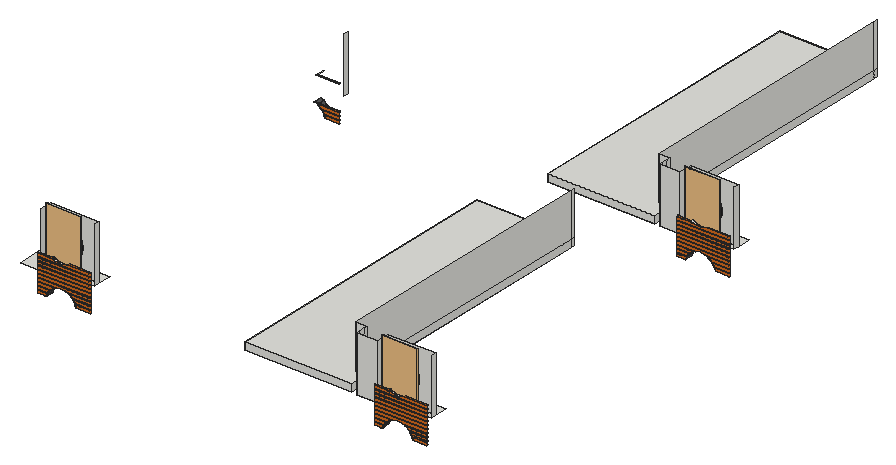
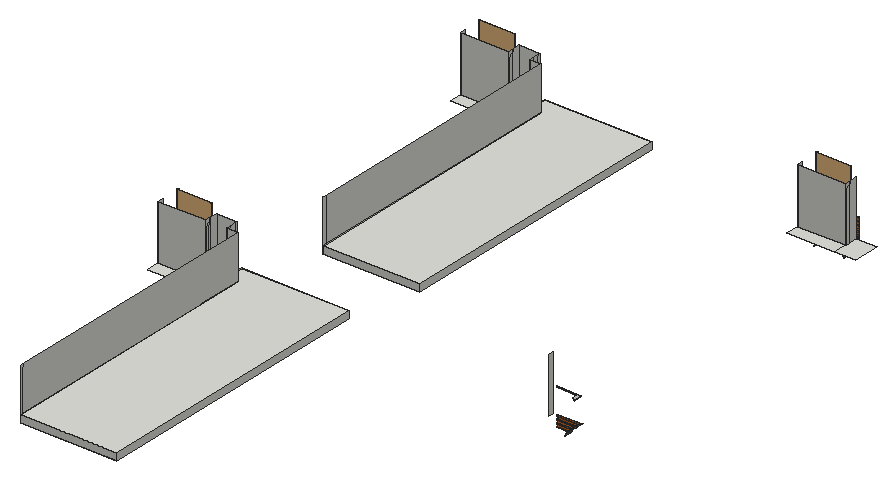
# SketchUp Ruby script. Lengths in inches.
U = 1.inch
M = Sketchup.active_model
def pt(a) = Geom::Point3d.new(a.map { |v| v * U })
def face(e, loops, mat)
  f = e.add_face(loops[0].map { |a| pt(a) })
  loops[1..].each { |l| e.add_face(l.map { |a| pt(a) }).erase! }
  f.material = f.back_material = mat if mat
  f
end
# faces: each face lists its corners as indices into pts; further lists are holes
def faces(e, pts, list, mat = nil) = list.each { |f| face(e, (f[0].is_a?(Array) ? f : [f]).map { |l| l.map { |i| pts[i] } }, mat) }
# xy, xz, yz: faces in a plane at the given z, y or x. An outline is a flat list of corners, or four numbers for a rectangle; further outlines are holes
def ring(l) = l.size == 4 ? [[l[0], l[1]], [l[2], l[1]], [l[2], l[3]], [l[0], l[3]]] : l.each_slice(2).to_a
def flat(e, list, mat, &to3) = list.each { |f| face(e, (f[0].is_a?(Array) ? f : [f]).map { |l| ring(l).map { |u, v| to3.(u, v) } }, mat) }
def xy(e, z, list, mat = nil) = flat(e, list, mat) { |x, y| [x, y, z] }
def xz(e, y, list, mat = nil) = flat(e, list, mat) { |x, z| [x, y, z] }
def yz(e, x, list, mat = nil) = flat(e, list, mat) { |y, z| [x, y, z] }
def lines(e, pts, list) = list.each { |a, b| e.add_line(pt(pts[a]), pt(pts[b])) }
# prism: a flat outline (further loops are holes) pulled along v
def prism(e, loops, v, mat = nil)
  f = face(e, loops, mat); d = Geom::Vector3d.new(v.map { |x| x * U })
  f.pushpull(f.normal.samedirection?(d) ? d.length : -d.length)
end
def box(e, o, s, mat = nil) = prism(e, [[o, [o[0] + s[0], o[1], o[2]], [o[0] + s[0], o[1] + s[1], o[2]], [o[0], o[1] + s[1], o[2]]]], [0, 0, s[2]], mat)
def at(x, y, z, deg = 0) = Geom::Transformation.translation(pt([x, y, z])) * Geom::Transformation.rotation(ORIGIN, Z_AXIS, deg.degrees)
def axes(o, x, y, z) = Geom::Transformation.new([*x, 0, *y, 0, *z, 0, *pt(o).to_a, 1])
def part(name) = M.definitions.add(name)
# library, detail: a bought-in or finely detailed component or shape, given as its bounding box
def library(name, o, s) = part(name).tap { |d| box(d.entities, o, s) }
def detail(e, o, s) = box(e.add_group.entities, o, s)
def put(e, d, t, mat = nil) = e.add_instance(d, t).tap { |i| i.material = mat if mat }
def group(e, t, mat = nil) = e.add_group.tap { |g| g.transformation = t; g.material = mat if mat }.entities
root = M.entities
M.materials.add("[0041_Chocolate]").color = [210, 105, 30]
M.materials.add("[Color M06]").color = [84, 84, 84]
M.materials.add("[Color M08]").color = [30, 30, 30]
c1 = library("1",[3.97,34.78,0],[101.43,33.99,0.79])
xy(root,260.375,[[1547.711,280.466,1564.025,281.466],[1621.742,280.466,1649.144,281.466],[2198.211,280.466,2214.525,281.466],[2272.242,280.466,2299.644,281.466],[1550.055,971.36,1577.456,972.36],
  [2230.648,971.36,2246.963,972.36],[2304.68,971.36,2332.081,972.36]],"[0041_Chocolate]")
xy(root,265.329,[[1547.711,280.466,1565.895,281.466],[1619.873,280.466,1649.144,281.466],[2198.211,280.466,2216.395,281.466],[2270.373,280.466,2299.644,281.466],[1548.185,971.36,1577.456,972.36],
  [2230.648,971.36,2248.832,972.36],[2302.81,971.36,2332.081,972.36]],"[0041_Chocolate]")
xy(root,267.4375,[[1547.711,280.466,1566.768,281.466],[1619,280.466,1649.144,281.466],[2198.211,280.466,2217.268,281.466],[2269.5,280.466,2299.644,281.466],[1547.312,971.36,1577.456,972.36],
  [2230.648,971.36,2249.705,972.36],[2301.937,971.36,2332.081,972.36]],"[0041_Chocolate]")
xy(root,272.392,[[1547.711,280.466,1570.298,281.466],[1615.47,280.466,1649.144,281.466],[2198.211,280.466,2220.798,281.466],[2265.97,280.466,2299.644,281.466],[1543.782,971.36,1577.456,972.36],
  [2230.648,971.36,2253.235,972.36],[2298.407,971.36,2332.081,972.36]],"[0041_Chocolate]")
xy(root,274.5,[[1547.711,280.466,1571.982,281.466],[1613.786,280.466,1649.144,281.466],[2198.211,280.466,2222.482,281.466],[2264.286,280.466,2299.644,281.466],[1542.098,971.36,1577.456,972.36],
  [2230.648,971.36,2254.92,972.36],[2296.723,971.36,2332.081,972.36]],"[0041_Chocolate]")
xy(root,279.454,[[1547.711,280.466,1578.821,281.466],[1606.946,280.466,1649.144,281.466],[2198.211,280.466,2229.321,281.466],[2257.446,280.466,2299.644,281.466],[1535.259,971.36,1577.456,972.36],
  [2230.648,971.36,2261.759,972.36],[2289.884,971.36,2332.081,972.36]],"[0041_Chocolate]")
xy(root,281.5625,[[1547.711,280.466,1583.911,281.466],[1601.857,280.466,1649.144,281.466],[2198.211,280.466,2234.411,281.466],[2252.357,280.466,2299.644,281.466],[1530.169,971.36,1577.456,972.36],
  [2230.648,971.36,2266.848,972.36],[2284.794,971.36,2332.081,972.36]],"[0041_Chocolate]")
xy(root,286.517,[[1547.711,280.466,1649.144,281.466],[2198.211,280.466,2299.644,281.466],[2230.648,971.36,2332.081,972.36]],"[0041_Chocolate]")
xy(root,288.625,[[1547.711,280.466,1649.144,281.466],[2198.211,280.466,2299.644,281.466],[2230.648,971.36,2332.081,972.36]],"[0041_Chocolate]")
xy(root,293.579,[[1547.711,280.466,1649.144,281.466],[2198.211,280.466,2299.644,281.466],[2230.648,971.36,2332.081,972.36]],"[0041_Chocolate]")
xy(root,295.6875,[[1547.711,280.466,1649.144,281.466],[2198.211,280.466,2299.644,281.466],[2230.648,971.36,2332.081,972.36]],"[0041_Chocolate]")
xy(root,295.724,[[1507.743,287.951,1547.711,337.5625],[2158.243,287.951,2198.211,337.5625],[1547.711,302.0625,1640.523,312.8125],[2198.211,302.0625,2291.023,312.8125],[1547.711,312.8125,1640.523,337.5625],
  [2198.211,312.8125,2291.023,337.5625],[2190.68,978.845,2230.648,1028.457],[2230.648,992.957,2323.461,1003.707],[2230.648,1003.707,2323.461,1028.457]])
xy(root,300.642,[[1547.711,280.466,1649.144,281.466],[2198.211,280.466,2299.644,281.466],[2230.648,971.36,2332.081,972.36]],"[0041_Chocolate]")
xy(root,302.75,[[1547.711,280.466,1649.144,281.466],[2198.211,280.466,2299.644,281.466],[2230.648,971.36,2332.081,972.36]],"[0041_Chocolate]")
xy(root,304.253,[[1949.897,277.25,1949.897,830.913,1958.44,830.913,1958.44,341.872,1958.689,338.079,1959.43,334.351,1960.652,330.752,1962.333,327.342,1963.672,325.339,1964.445,324.182,1965.225,323.293,1966.952,321.324,1969.809,318.818,1972.97,316.706,1976.379,315.025,1979.979,313.803,1983.707,313.061,1987.5,312.8125,2157.378,312.8125,2157.378,277.25],[1987.5,312.8125,2137.003,312.8125,2137.003,325.339,1993.245,325.339,1989.587,325.579,1985.993,326.294,1982.522,327.472,1979.235,329.093,1976.187,331.129,1973.432,333.546,1971.015,336.301,1968.979,339.349,1967.358,342.636,1966.179,346.107,1965.464,349.702,1965.225,353.359,1965.225,323.293,1966.952,321.324,1969.809,318.818,1972.97,316.706,1976.379,315.025,1979.979,313.803,1983.707,313.061],[1965.225,323.293,1965.225,830.913,1958.44,830.913,1958.44,341.872,1958.689,338.079,1959.43,334.351,1960.652,330.752,1962.333,327.342,1963.672,325.339,1964.445,324.182],[1993.245,325.339,1989.587,325.579,1985.993,326.294,1982.522,327.472,1979.235,329.093,1976.187,331.129,1973.432,333.546,1971.015,336.301,1968.979,339.349,1967.358,342.636,1966.179,346.107,1965.464,349.702,1965.225,353.359,1965.225,830.913,2137.003,830.913,2137.003,325.339],[1949.897,830.913,2137.003,838.144],
  [1982.334,968.144,1982.334,1521.808,1990.878,1521.808,1990.878,1032.767,1991.126,1028.973,1991.868,1025.245,1993.09,1021.646,1994.771,1018.237,1996.11,1016.233,1996.883,1015.076,1997.662,1014.187,1999.389,1012.218,2002.247,1009.712,2005.407,1007.6,2008.817,1005.919,2012.416,1004.697,2016.144,1003.955,2019.9375,1003.707,2189.815,1003.707,2189.815,968.144],[2019.9375,1003.707,2169.44,1003.707,2169.44,1016.233,2025.682,1016.233,2022.025,1016.473,2018.43,1017.188,2014.959,1018.366,2011.672,1019.987,2008.625,1022.023,2005.869,1024.44,2003.452,1027.196,2001.416,1030.243,1999.795,1033.53,1998.617,1037.001,1997.902,1040.596,1997.662,1044.253,1997.662,1014.187,1999.389,1012.218,2002.247,1009.712,2005.407,1007.6,2008.817,1005.919,2012.416,1004.697,2016.144,1003.955],[1997.662,1014.187,1997.662,1521.808,1990.878,1521.808,1990.878,1032.767,1991.126,1028.973,1991.868,1025.245,1993.09,1021.646,1994.771,1018.237,1996.11,1016.233,1996.883,1015.076],[2025.682,1016.233,2022.025,1016.473,2018.43,1017.188,2014.959,1018.366,2011.672,1019.987,2008.625,1022.023,2005.869,1024.44,2003.452,1027.196,2001.416,1030.243,1999.795,1033.53,1998.617,1037.001,1997.902,1040.596,1997.662,1044.253,1997.662,1521.808,2169.44,1521.808,2169.44,1016.233],[1982.334,1521.808,2169.44,1529.038]])
xy(root,307.704,[[1547.711,280.466,1649.144,281.466],[2198.211,280.466,2299.644,281.466],[2230.648,971.36,2332.081,972.36]],"[0041_Chocolate]")
xy(root,309.8125,[[1547.711,280.466,1649.144,281.466],[2198.211,280.466,2299.644,281.466],[2230.648,971.36,2332.081,972.36]],"[0041_Chocolate]")
xy(root,314.767,[[1547.711,280.466,1649.144,281.466],[2198.211,280.466,2299.644,281.466],[2230.648,971.36,2332.081,972.36]],"[0041_Chocolate]")
xy(root,316.875,[[1547.711,280.466,1649.144,281.466],[2198.211,280.466,2299.644,281.466],[2230.648,971.36,2332.081,972.36]],"[0041_Chocolate]")
xy(root,318.066,[[1949.897,277.25,2157.378,277.25,2157.378,312.8125,2137.003,312.8125,2137.003,838.144,1949.897,838.144],[1982.334,968.144,2189.815,968.144,2189.815,1003.707,2169.44,1003.707,2169.44,1529.038,1982.334,1529.038]])
xy(root,321.829,[[1547.711,280.466,1649.144,281.466],[2198.211,280.466,2299.644,281.466],[2230.648,971.36,2332.081,972.36]],"[0041_Chocolate]")
xy(root,323.9375,[[1547.711,280.466,1649.144,281.466],[2198.211,280.466,2299.644,281.466],[2230.648,971.36,2332.081,972.36]],"[0041_Chocolate]")
xy(root,328.892,[[1547.711,280.466,1577.856,281.466],[1604.375,280.466,1649.144,281.466],[2198.211,280.466,2228.356,281.466],[2254.875,280.466,2299.644,281.466],[1532.6875,971.36,1577.456,972.36],
  [2230.648,971.36,2260.794,972.36],[2287.3125,971.36,2332.081,972.36]],"[0041_Chocolate]")
xz(root,277.25,[[1949.897,304.253,2157.378,318.066]])
xz(root,280.466,[[1547.711,260.375,1564.025,260.375,1564.111,261.022,1565.895,265.329,1547.711,265.329],[1621.742,260.375,1649.144,260.375,1649.144,265.329,1619.873,265.329,1621.657,261.022],[2198.211,260.375,2214.525,260.375,2214.611,261.022,2216.395,265.329,2198.211,265.329],[2272.242,260.375,2299.644,260.375,2299.644,265.329,2270.373,265.329,2272.157,261.022],[1547.711,267.4375,1566.768,267.4375,1567.086,268.207,1570.298,272.392,1547.711,272.392],
  [1619,267.4375,1649.144,267.4375,1649.144,272.392,1615.47,272.392,1618.681,268.207],[2198.211,267.4375,2217.268,267.4375,2217.586,268.207,2220.798,272.392,2198.211,272.392],[2269.5,267.4375,2299.644,267.4375,2299.644,272.392,2265.97,272.392,2269.181,268.207],[1547.711,274.5,1571.982,274.5,1577.99,279.11,1578.821,279.454,1547.711,279.454],[1613.786,274.5,1649.144,274.5,1649.144,279.454,1606.946,279.454,1607.778,279.11],
  [2198.211,274.5,2222.482,274.5,2228.49,279.11,2229.321,279.454,2198.211,279.454],[2264.286,274.5,2299.644,274.5,2299.644,279.454,2257.446,279.454,2258.278,279.11],[1547.711,281.5625,1583.911,281.5625,1585.174,282.086,1592.884,283.101,1600.594,282.086,1601.857,281.5625,1649.144,281.5625,1649.144,286.517,1547.711,286.517],[2198.211,281.5625,2234.411,281.5625,2235.674,282.086,2243.384,283.101,2251.094,282.086,2252.357,281.5625,2299.644,281.5625,2299.644,286.517,2198.211,286.517],[1547.711,288.625,1649.144,293.579],
  [2198.211,288.625,2299.644,293.579],[1547.711,295.6875,1649.144,300.642],[2198.211,295.6875,2299.644,300.642],[1547.711,302.75,1649.144,307.704],[2198.211,302.75,2299.644,307.704],
  [1547.711,309.8125,1649.144,314.767],[2198.211,309.8125,2299.644,314.767],[1547.711,316.875,1649.144,321.829],[2198.211,316.875,2299.644,321.829],[1547.711,323.9375,1649.144,323.9375,1649.144,328.892,1604.375,328.892,1603.131,328.172,1595.223,326.049,1587.036,326.045,1579.126,328.16,1577.856,328.892,1547.711,328.892],
  [2198.211,323.9375,2299.644,323.9375,2299.644,328.892,2254.875,328.892,2253.631,328.172,2245.723,326.049,2237.536,326.045,2229.626,328.16,2228.356,328.892,2198.211,328.892]],"[0041_Chocolate]")
xz(root,281.466,[[1547.711,265.329,1565.895,265.329,1566.768,267.4375,1547.711,267.4375],[1619.873,265.329,1649.144,265.329,1649.144,267.4375,1619,267.4375],[2198.211,265.329,2216.395,265.329,2217.268,267.4375,2198.211,267.4375],[2270.373,265.329,2299.644,265.329,2299.644,267.4375,2269.5,267.4375],[1547.711,272.392,1570.298,272.392,1571.82,274.376,1571.982,274.5,1547.711,274.5],
  [1615.47,272.392,1649.144,272.392,1649.144,274.5,1613.786,274.5,1613.947,274.376],[2198.211,272.392,2220.798,272.392,2222.32,274.376,2222.482,274.5,2198.211,274.5],[2265.97,272.392,2299.644,272.392,2299.644,274.5,2264.286,274.5,2264.447,274.376],[1547.711,279.454,1578.821,279.454,1583.911,281.5625,1547.711,281.5625],[1606.946,279.454,1649.144,279.454,1649.144,281.5625,1601.857,281.5625],
  [2198.211,279.454,2229.321,279.454,2234.411,281.5625,2198.211,281.5625],[2257.446,279.454,2299.644,279.454,2299.644,281.5625,2252.357,281.5625],[1547.711,286.517,1649.144,288.625],[2198.211,286.517,2299.644,288.625],[1547.711,293.579,1649.144,295.6875],
  [2198.211,293.579,2299.644,295.6875],[1547.711,300.642,1649.144,302.75],[2198.211,300.642,2299.644,302.75],[1547.711,307.704,1649.144,309.8125],[2198.211,307.704,2299.644,309.8125],
  [1547.711,314.767,1649.144,316.875],[2198.211,314.767,2299.644,316.875],[1547.711,321.829,1649.144,323.9375],[2198.211,321.829,2299.644,323.9375],[1547.711,328.892,1577.856,328.892,1574.2,331,1547.711,331],
  [1604.375,328.892,1649.144,328.892,1649.144,331,1608.022,331],[2198.211,328.892,2228.356,328.892,2224.7,331,2198.211,331],[2254.875,328.892,2299.644,328.892,2299.644,331,2258.522,331]],"[0041_Chocolate]")
xz(root,287.951,[[2158.243,295.724,2198.211,402.635]])
xz(root,295.653,[[1587.036,326.045,1595.223,326.049,1603.131,328.172,1604.375,328.892,1608.022,331,1610.219,332.27,1613.899,335.954,1616.005,338.0625,1618.862,343.017,1620.078,345.125,1620.095,345.155,1621.412,350.079,1621.975,352.1875,1622.21,353.065,1622.208,357.142,1622.207,359.25,1622.206,361.252,1621.413,364.204,1620.847,366.3125,1620.082,369.16,1618.864,371.267,1617.754,373.1875,1615.985,376.248,1614.089,378.142,1612.166,380.0625,1610.192,382.034,1605.02,385.017,1603.099,386.124,1600.057,386.9375,1595.19,388.239,1587.002,388.234,1582.173,386.9375,1579.095,386.111,1577.202,385.017,1572.007,382.014,1570.058,380.0625,1568.139,378.142,1566.221,376.221,1564.471,373.1875,1563.364,371.267,1562.131,369.128,1561.378,366.3125,1560.814,364.204,1560.016,361.219,1560.017,359.25,1560.018,357.142,1560.02,353.031,1560.247,352.1875,1560.813,350.079,1562.143,345.125,1562.144,345.124,1563.362,343.017,1566.226,338.0625,1566.241,338.036,1568.325,335.954,1572.034,332.249,1574.2,331,1577.856,328.892,1579.126,328.16],[2237.536,326.045,2245.723,326.049,2253.631,328.172,2254.875,328.892,2258.522,331,2260.719,332.27,2264.399,335.954,2266.505,338.0625,2269.362,343.017,2270.578,345.125,2270.595,345.155,2271.912,350.079,2272.475,352.1875,2272.71,353.065,2272.708,357.142,2272.707,359.25,2272.706,361.252,2271.913,364.204,2271.347,366.3125,2270.582,369.16,2269.364,371.267,2268.254,373.1875,2266.485,376.248,2264.589,378.142,2262.666,380.0625,2260.692,382.034,2255.52,385.017,2253.599,386.124,2250.557,386.9375,2245.69,388.239,2237.502,388.234,2232.673,386.9375,2229.595,386.111,2227.702,385.017,2222.507,382.014,2220.558,380.0625,2218.639,378.142,2216.721,376.221,2214.971,373.1875,2213.864,371.267,2212.631,369.128,2211.878,366.3125,2211.314,364.204,2210.516,361.219,2210.517,359.25,2210.518,357.142,2210.52,353.031,2210.747,352.1875,2211.313,350.079,2212.643,345.125,2212.644,345.124,2213.862,343.017,2216.726,338.0625,2216.741,338.036,2218.825,335.954,2222.534,332.249,2224.7,331,2228.356,328.892,2229.626,328.16]],"[Color M08]")
xz(root,312.8125,[[1547.711,295.724,1640.523,402.635],[2198.211,295.724,2291.023,402.635],[2137.003,304.253,2157.378,318.066],[2157.378,304.253,2158.243,309.691],[2157.378,309.691,2158.243,309.691,2158.243,402.635,2137.003,402.635,2137.003,318.066,2157.378,318.066]])
xz(root,838.144,[[1949.897,304.253,2137.003,318.066]])
xz(root,968.144,[[1982.334,304.253,2189.815,318.066]])
xz(root,971.36,[[1550.055,260.375,1577.456,260.375,1577.456,265.329,1548.185,265.329,1549.969,261.022],[2230.648,260.375,2246.963,260.375,2247.048,261.022,2248.832,265.329,2230.648,265.329],[2304.68,260.375,2332.081,260.375,2332.081,265.329,2302.81,265.329,2304.594,261.022],[1547.312,267.4375,1577.456,267.4375,1577.456,272.392,1543.782,272.392,1546.994,268.207],[2230.648,267.4375,2249.705,267.4375,2250.024,268.207,2253.235,272.392,2230.648,272.392],
  [2301.937,267.4375,2332.081,267.4375,2332.081,272.392,2298.407,272.392,2301.619,268.207],[1542.098,274.5,1577.456,274.5,1577.456,279.454,1535.259,279.454,1536.09,279.11],[2230.648,274.5,2254.92,274.5,2260.927,279.11,2261.759,279.454,2230.648,279.454],[2296.723,274.5,2332.081,274.5,2332.081,279.454,2289.884,279.454,2290.715,279.11],[2230.648,281.5625,2266.848,281.5625,2268.112,282.086,2275.821,283.101,2283.531,282.086,2284.794,281.5625,2332.081,281.5625,2332.081,286.517,2230.648,286.517],
  [2230.648,288.625,2332.081,293.579],[2230.648,295.6875,2332.081,300.642],[2230.648,302.75,2332.081,307.704],[2230.648,309.8125,2332.081,314.767],[2230.648,316.875,2332.081,321.829],
  [2230.648,323.9375,2332.081,323.9375,2332.081,328.892,2287.3125,328.892,2286.068,328.172,2278.161,326.049,2269.973,326.045,2262.064,328.16,2260.794,328.892,2230.648,328.892]],"[0041_Chocolate]")
xz(root,972.36,[[1548.185,265.329,1577.456,265.329,1577.456,267.4375,1547.312,267.4375],[2230.648,265.329,2248.832,265.329,2249.705,267.4375,2230.648,267.4375],[2302.81,265.329,2332.081,265.329,2332.081,267.4375,2301.937,267.4375],[1543.782,272.392,1577.456,272.392,1577.456,274.5,1542.098,274.5,1542.26,274.376],[2230.648,272.392,2253.235,272.392,2254.758,274.376,2254.92,274.5,2230.648,274.5],
  [2298.407,272.392,2332.081,272.392,2332.081,274.5,2296.723,274.5,2296.885,274.376],[1535.259,279.454,1577.456,279.454,1577.456,281.5625,1530.169,281.5625],[2230.648,279.454,2261.759,279.454,2266.848,281.5625,2230.648,281.5625],[2289.884,279.454,2332.081,279.454,2332.081,281.5625,2284.794,281.5625],[2230.648,286.517,2332.081,288.625],
  [2230.648,293.579,2332.081,295.6875],[2230.648,300.642,2332.081,302.75],[2230.648,307.704,2332.081,309.8125],[2230.648,314.767,2332.081,316.875],[2230.648,321.829,2332.081,323.9375],
  [1532.6875,328.892,1577.456,328.892,1577.456,331,1536.335,331],[2230.648,328.892,2260.794,328.892,2257.138,331,2230.648,331],[2287.3125,328.892,2332.081,328.892,2332.081,331,2290.96,331]],"[0041_Chocolate]")
xz(root,978.845,[[2190.68,295.724,2230.648,402.635]])
xz(root,986.548,[[2269.973,326.045,2278.161,326.049,2286.068,328.172,2287.3125,328.892,2290.96,331,2293.157,332.27,2296.837,335.954,2298.943,338.0625,2301.8,343.017,2303.015,345.125,2303.033,345.155,2304.349,350.079,2304.913,352.1875,2305.147,353.065,2305.145,357.142,2305.144,359.25,2305.143,361.252,2304.35,364.204,2303.784,366.3125,2303.02,369.16,2301.802,371.267,2300.691,373.1875,2298.922,376.248,2297.026,378.142,2295.103,380.0625,2293.13,382.034,2287.957,385.017,2286.037,386.124,2282.995,386.9375,2278.127,388.239,2269.94,388.234,2265.11,386.9375,2262.033,386.111,2260.14,385.017,2254.944,382.014,2252.995,380.0625,2251.077,378.142,2249.158,376.221,2247.409,373.1875,2246.301,371.267,2245.068,369.128,2244.315,366.3125,2243.752,364.204,2242.953,361.219,2242.954,359.25,2242.956,357.142,2242.958,353.031,2243.184,352.1875,2243.75,350.079,2245.081,345.125,2245.081,345.124,2246.299,343.017,2249.163,338.0625,2249.179,338.036,2251.262,335.954,2254.971,332.249,2257.138,331,2260.794,328.892,2262.064,328.16]],"[Color M08]")
xz(root,1003.707,[[2230.648,295.724,2323.461,402.635],[2169.44,304.253,2189.815,318.066],[2189.815,304.253,2190.68,309.691],[2189.815,309.691,2190.68,309.691,2190.68,402.635,2169.44,402.635,2169.44,318.066,2189.815,318.066]])
xz(root,1529.038,[[1982.334,304.253,2169.44,318.066]])
yz(root,1547.711,[[287.951,295.724,302.457,295.724,302.457,395.26,300.332,395.26,300.332,402.635,287.951,402.635],[302.457,295.724,305.582,395.26],[305.582,295.724,310.269,395.26],[310.269,295.724,312.8125,295.724,312.8125,402.635,305.582,402.635,305.582,395.26,310.269,395.26]])
yz(root,1568.836,[[993.351,295.724,1003.707,402.635]])
yz(root,1640.523,[[302.457,295.724,312.8125,402.635]])
yz(root,1949.897,[[277.25,304.253,838.144,318.066]])
yz(root,1982.334,[[968.144,304.253,1529.038,318.066]])
yz(root,2137.003,[[312.8125,304.253,397.858,318.066],[397.858,304.253,406.382,318.066],[406.382,304.253,830.913,318.066],[830.913,304.253,838.144,318.066],[312.8125,318.066,830.913,402.635],
  [830.913,318.066,838.144,402.635]])
yz(root,2157.378,[[277.25,304.253,312.8125,318.066]])
yz(root,2158.243,[[287.951,295.724,292.451,304.253],[292.451,295.724,305.582,304.253],[305.582,295.724,312.8125,304.253],[287.951,304.253,292.451,309.691],[292.451,304.253,305.582,309.691],
  [305.582,304.253,312.8125,309.691],[287.951,309.691,292.451,402.635],[292.451,309.691,305.582,402.635],[305.582,309.691,312.8125,402.635]])
yz(root,2169.44,[[1003.707,304.253,1088.752,318.066],[1088.752,304.253,1097.276,318.066],[1097.276,304.253,1521.808,318.066],[1521.808,304.253,1529.038,318.066],[1003.707,318.066,1521.808,402.635],
  [1521.808,318.066,1529.038,402.635]])
yz(root,2189.815,[[968.144,304.253,1003.707,318.066]])
yz(root,2190.68,[[978.845,295.724,983.345,304.253],[983.345,295.724,996.476,304.253],[996.476,295.724,1003.707,304.253],[978.845,304.253,983.345,309.691],[983.345,304.253,996.476,309.691],
  [996.476,304.253,1003.707,309.691],[978.845,309.691,983.345,402.635],[983.345,309.691,996.476,402.635],[996.476,309.691,1003.707,402.635]])
yz(root,2198.211,[[287.951,295.724,302.457,295.724,302.457,395.26,300.332,395.26,300.332,402.635,287.951,402.635],[302.457,295.724,305.582,395.26],[305.582,295.724,310.269,395.26],[310.269,295.724,312.8125,295.724,312.8125,402.635,305.582,402.635,305.582,395.26,310.269,395.26]])
yz(root,2230.648,[[978.845,295.724,993.351,295.724,993.351,395.26,991.226,395.26,991.226,402.635,978.845,402.635],[993.351,295.724,996.476,395.26],[1001.163,295.724,1003.707,295.724,1003.707,402.635,996.476,402.635,996.476,395.26,1001.163,395.26],[996.476,295.724,1001.163,395.26]])
yz(root,2291.023,[[302.457,295.724,312.8125,402.635]])
yz(root,2323.461,[[993.351,295.724,1003.707,402.635]])
p = [[1564.111,295.653,261.022],[1564.111,280.466,261.022],[1564.025,280.466,260.375],[1564.025,281.466,260.375],[1564.025,295.653,260.375],[1621.742,295.653,260.375],
  [1621.742,281.466,260.375],[1621.742,280.466,260.375],[1621.657,280.466,261.022],[1621.657,295.653,261.022],[2214.611,295.653,261.022],[2214.611,280.466,261.022],
  [2214.525,280.466,260.375],[2214.525,281.466,260.375],[2214.525,295.653,260.375],[2272.242,295.653,260.375],[2272.242,281.466,260.375],[2272.242,280.466,260.375],
  [2272.157,280.466,261.022],[2272.157,295.653,261.022],[1550.055,986.548,260.375],[1550.055,972.36,260.375],[1550.055,971.36,260.375],[1549.969,971.36,261.022],
  [1549.969,986.548,261.022],[2247.048,986.548,261.022],[2247.048,971.36,261.022],[2246.963,971.36,260.375],[2246.963,972.36,260.375],[2246.963,986.548,260.375],
  [2304.68,986.548,260.375],[2304.68,972.36,260.375],[2304.68,971.36,260.375],[2304.594,971.36,261.022],[2304.594,986.548,261.022],[1565.895,295.653,265.329],
  [1565.895,281.466,265.329],[1565.895,280.466,265.329],[1619.873,280.466,265.329],[1619.873,281.466,265.329],[1619.873,295.653,265.329],[2216.395,295.653,265.329],
  [2216.395,281.466,265.329],[2216.395,280.466,265.329],[2270.373,280.466,265.329],[2270.373,281.466,265.329],[2270.373,295.653,265.329],[1548.185,971.36,265.329],
  [1548.185,972.36,265.329],[1548.185,986.548,265.329],[2248.832,986.548,265.329],[2248.832,972.36,265.329],[2248.832,971.36,265.329],[2302.81,971.36,265.329],
  [2302.81,972.36,265.329],[2302.81,986.548,265.329],[1566.768,281.466,267.4375],[1566.768,295.653,267.4375],[1619,281.466,267.4375],[1619,295.653,267.4375],
  [2217.268,281.466,267.4375],[2217.268,295.653,267.4375],[2269.5,281.466,267.4375],[2269.5,295.653,267.4375],[1547.312,972.36,267.4375],[1547.312,986.548,267.4375],
  [2249.705,972.36,267.4375],[2249.705,986.548,267.4375],[2301.937,972.36,267.4375],[2301.937,986.548,267.4375],[1567.086,295.653,268.207],[1567.086,280.466,268.207],
  [1566.768,280.466,267.4375],[1619,280.466,267.4375],[1618.681,280.466,268.207],[1618.681,295.653,268.207],[2217.586,295.653,268.207],[2217.586,280.466,268.207],
  [2217.268,280.466,267.4375],[2269.5,280.466,267.4375],[2269.181,280.466,268.207],[2269.181,295.653,268.207],[1547.312,971.36,267.4375],[1546.994,971.36,268.207],
  [1546.994,986.548,268.207],[2250.024,986.548,268.207],[2250.024,971.36,268.207],[2249.705,971.36,267.4375],[2301.937,971.36,267.4375],[2301.619,971.36,268.207],
  [2301.619,986.548,268.207],[1570.298,295.653,272.392],[1570.298,281.466,272.392],[1570.298,280.466,272.392],[1615.47,280.466,272.392],[1615.47,281.466,272.392],
  [1615.47,295.653,272.392],[2220.798,295.653,272.392],[2220.798,281.466,272.392],[2220.798,280.466,272.392],[2265.97,280.466,272.392],[2265.97,281.466,272.392],
  [2265.97,295.653,272.392],[1543.782,971.36,272.392],[1543.782,972.36,272.392],[1543.782,986.548,272.392],[2253.235,986.548,272.392],[2253.235,972.36,272.392],
  [2253.235,971.36,272.392],[2298.407,971.36,272.392],[2298.407,972.36,272.392],[2298.407,986.548,272.392],[1571.82,281.466,274.376],[1571.82,295.653,274.376],
  [1613.947,281.466,274.376],[1613.947,295.653,274.376],[2222.32,281.466,274.376],[2222.32,295.653,274.376],[2264.447,281.466,274.376],[2264.447,295.653,274.376],
  [1542.26,972.36,274.376],[1542.26,986.548,274.376],[2254.758,972.36,274.376],[2254.758,986.548,274.376],[2296.885,972.36,274.376],[2296.885,986.548,274.376],
  [1571.982,281.466,274.5],[1571.982,295.653,274.5],[1613.786,281.466,274.5],[1613.786,295.653,274.5],[2222.482,281.466,274.5],[2222.482,295.653,274.5],
  [2264.286,281.466,274.5],[2264.286,295.653,274.5],[1542.098,972.36,274.5],[1542.098,986.548,274.5],[2254.92,972.36,274.5],[2254.92,986.548,274.5],
  [2296.723,972.36,274.5],[2296.723,986.548,274.5],[1577.99,295.653,279.11],[1577.99,280.466,279.11],[1571.982,280.466,274.5],[1613.786,280.466,274.5],
  [1607.778,280.466,279.11],[1607.778,295.653,279.11],[2228.49,295.653,279.11],[2228.49,280.466,279.11],[2222.482,280.466,274.5],[2264.286,280.466,274.5],
  [2258.278,280.466,279.11],[2258.278,295.653,279.11],[1542.098,971.36,274.5],[1536.09,971.36,279.11],[1536.09,986.548,279.11],[2260.927,986.548,279.11],
  [2260.927,971.36,279.11],[2254.92,971.36,274.5],[2296.723,971.36,274.5],[2290.715,971.36,279.11],[2290.715,986.548,279.11],[1578.821,295.653,279.454],
  [1578.821,281.466,279.454],[1578.821,280.466,279.454],[1606.946,280.466,279.454],[1606.946,281.466,279.454],[1606.946,295.653,279.454],[2229.321,295.653,279.454],
  [2229.321,281.466,279.454],[2229.321,280.466,279.454],[2257.446,280.466,279.454],[2257.446,281.466,279.454],[2257.446,295.653,279.454],[1535.259,971.36,279.454],
  [1535.259,972.36,279.454],[1535.259,986.548,279.454],[2261.759,986.548,279.454],[2261.759,972.36,279.454],[2261.759,971.36,279.454],[2289.884,971.36,279.454],
  [2289.884,972.36,279.454],[2289.884,986.548,279.454],[1583.911,281.466,281.5625],[1583.911,295.653,281.5625],[1601.857,281.466,281.5625],[1601.857,295.653,281.5625],
  [2234.411,281.466,281.5625],[2234.411,295.653,281.5625],[2252.357,281.466,281.5625],[2252.357,295.653,281.5625],[1530.169,972.36,281.5625],[1530.169,986.548,281.5625],
  [2266.848,972.36,281.5625],[2266.848,986.548,281.5625],[2284.794,972.36,281.5625],[2284.794,986.548,281.5625],[1585.174,295.653,282.086],[1585.174,280.466,282.086],
  [1583.911,280.466,281.5625],[1601.857,280.466,281.5625],[1600.594,280.466,282.086],[1600.594,295.653,282.086],[2235.674,295.653,282.086],[2235.674,280.466,282.086],
  [2234.411,280.466,281.5625],[2252.357,280.466,281.5625],[2251.094,280.466,282.086],[2251.094,295.653,282.086],[1530.169,971.36,281.5625],[1528.906,971.36,282.086],
  [1528.906,986.548,282.086],[2268.112,986.548,282.086],[2268.112,971.36,282.086],[2266.848,971.36,281.5625],[2284.794,971.36,281.5625],[2283.531,971.36,282.086],
  [2283.531,986.548,282.086],[1592.884,295.653,283.101],[1592.884,280.466,283.101],[2243.384,295.653,283.101],[2243.384,280.466,283.101],[2275.821,986.548,283.101],
  [2275.821,971.36,283.101],[1579.126,295.653,328.16],[1579.126,280.466,328.16],[1587.036,280.466,326.045],[1587.036,295.653,326.045],[1595.223,280.466,326.049],
  [1595.223,295.653,326.049],[1603.131,280.466,328.172],[1603.131,295.653,328.172],[2229.626,295.653,328.16],[2229.626,280.466,328.16],[2237.536,280.466,326.045],
  [2237.536,295.653,326.045],[2245.723,280.466,326.049],[2245.723,295.653,326.049],[2253.631,280.466,328.172],[2253.631,295.653,328.172],[2262.064,986.548,328.16],
  [2262.064,971.36,328.16],[2269.973,971.36,326.045],[2269.973,986.548,326.045],[2278.161,971.36,326.049],[2278.161,986.548,326.049],[2286.068,971.36,328.172],
  [2286.068,986.548,328.172],[1577.856,295.653,328.892],[1577.856,281.466,328.892],[1577.856,280.466,328.892],[1604.375,280.466,328.892],[1604.375,281.466,328.892],
  [1604.375,295.653,328.892],[2228.356,295.653,328.892],[2228.356,281.466,328.892],[2228.356,280.466,328.892],[2254.875,280.466,328.892],[2254.875,281.466,328.892],
  [2254.875,295.653,328.892],[1531.443,986.548,328.172],[1531.443,971.36,328.172],[1532.6875,971.36,328.892],[1532.6875,972.36,328.892],[1532.6875,986.548,328.892],
  [2260.794,986.548,328.892],[2260.794,972.36,328.892],[2260.794,971.36,328.892],[2287.3125,971.36,328.892],[2287.3125,972.36,328.892],[2287.3125,986.548,328.892],
  [1574.2,281.466,331],[1574.2,295.653,331],[1608.022,281.466,331],[1608.022,295.653,331],[2224.7,281.466,331],[2224.7,295.653,331],
  [2258.522,281.466,331],[2258.522,295.653,331],[1536.335,972.36,331],[1536.335,986.548,331],[2257.138,972.36,331],[2257.138,986.548,331],
  [2290.96,972.36,331],[2290.96,986.548,331]]
faces(root,p,[[0,1,2,3,4],[5,6,7,8,9],[10,11,12,13,14],[15,16,17,18,19],[20,21,22,23,24],[25,26,27,28,29],[30,31,32,33,34],[35,36,37,1,0],
  [9,8,38,39,40],[41,42,43,11,10],[19,18,44,45,46],[24,23,47,48,49],[50,51,52,26,25],[34,33,53,54,55],[56,36,35,57],[39,58,59,40],
  [60,42,41,61],[45,62,63,46],[48,64,65,49],[66,51,50,67],[54,68,69,55],[70,71,72,56,57],[59,58,73,74,75],[76,77,78,60,61],
  [63,62,79,80,81],[65,64,82,83,84],[85,86,87,66,67],[69,68,88,89,90],[91,92,93,71,70],[75,74,94,95,96],[97,98,99,77,76],[81,80,100,101,102],
  [84,83,103,104,105],[106,107,108,86,85],[90,89,109,110,111],[112,92,91,113],[95,114,115,96],[116,98,97,117],[101,118,119,102],[104,120,121,105],
  [122,107,106,123],[110,124,125,111],[126,112,113,127],[114,128,129,115],[130,116,117,131],[118,132,133,119],[120,134,135,121],[136,122,123,137],
  [124,138,139,125],[140,141,142,126,127],[129,128,143,144,145],[146,147,148,130,131],[133,132,149,150,151],[135,134,152,153,154],[155,156,157,136,137],[139,138,158,159,160],
  [161,162,163,141,140],[145,144,164,165,166],[167,168,169,147,146],[151,150,170,171,172],[154,153,173,174,175],[176,177,178,156,155],[160,159,179,180,181],[182,162,161,183],
  [165,184,185,166],[186,168,167,187],[171,188,189,172],[174,190,191,175],[192,177,176,193],[180,194,195,181],[196,197,198,182,183],[185,184,199,200,201],
  [202,203,204,186,187],[189,188,205,206,207],[191,190,208,209,210],[211,212,213,192,193],[195,194,214,215,216],[217,218,197,196],[201,200,218,217],[219,220,203,202],
  [207,206,220,219],[221,222,212,211],[216,215,222,221]],"[Color M06]")
faces(root,p,[[223,224,225,226],[226,225,227,228],[228,227,229,230],[231,232,233,234],[234,233,235,236],[236,235,237,238],[239,240,241,242],[242,241,243,244],
  [244,243,245,246],[247,248,249,224,223],[230,229,250,251,252],[253,254,255,232,231],[238,237,256,257,258],[259,260,261,262,263],[264,265,266,240,239],[246,245,267,268,269],
  [270,248,247,271],[251,272,273,252],[274,254,253,275],[257,276,277,258],[262,278,279,263],[280,265,264,281],[268,282,283,269]])
put(root,c1,axes([1695.77,286.15,312.08],[0,0,1],[-2,0,0],[0,-1,0]))
put(root,c1,axes([2346.27,286.15,312.08],[0,0,1],[-2,0,0],[0,-1,0]))
put(root,c1,axes([2378.71,977.04,312.08],[0,0,1],[-2,0,0],[0,-1,0]))
